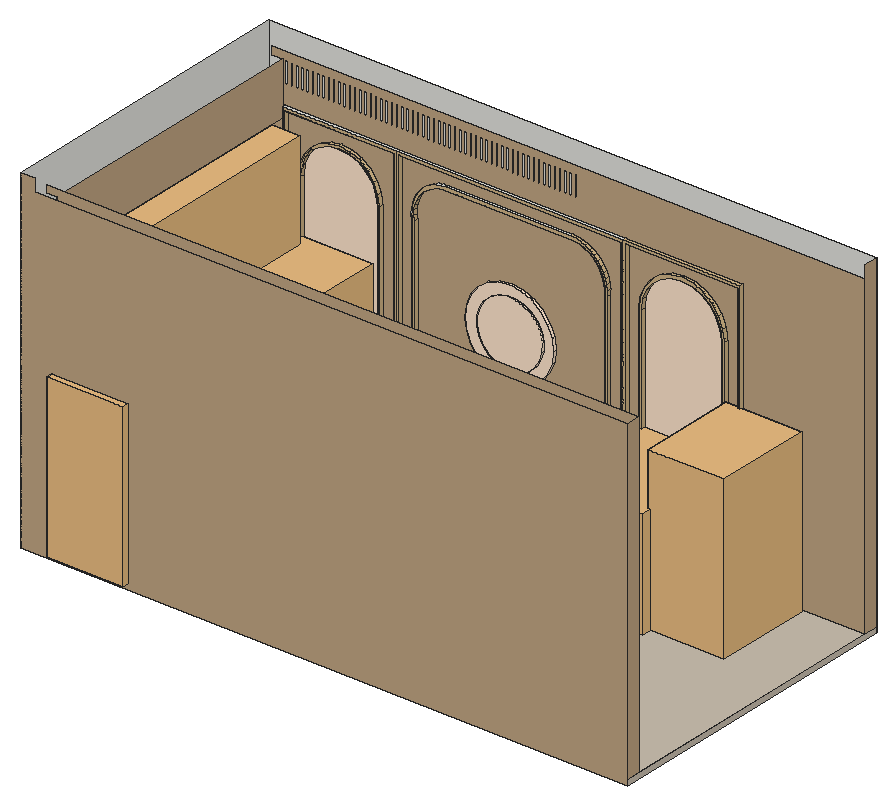
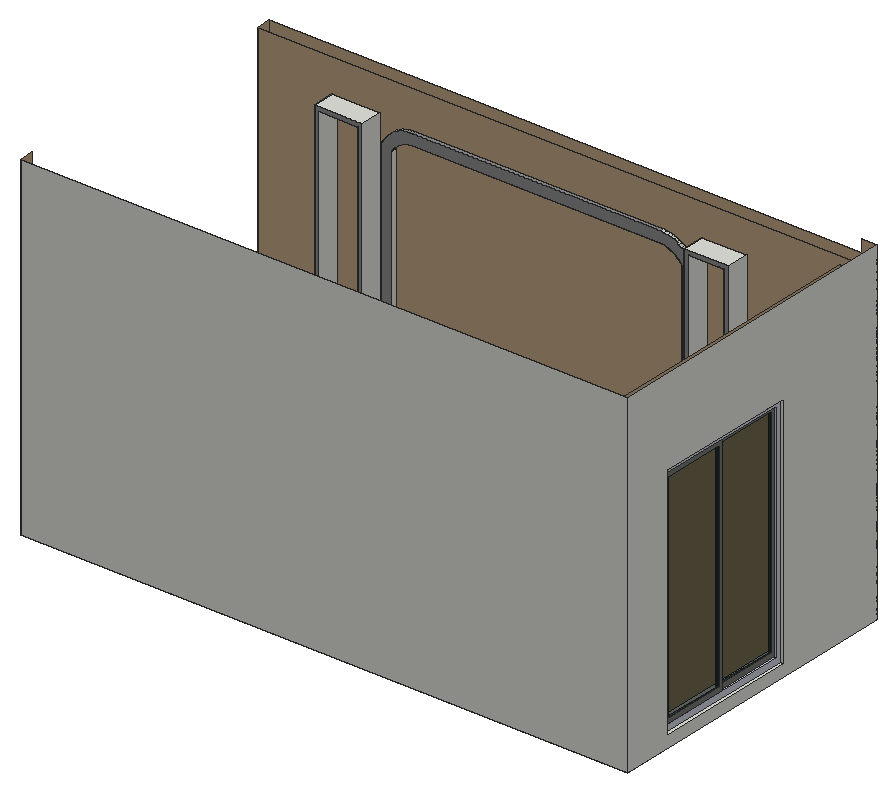
# SketchUp Ruby script. Lengths in inches.
U = 1.inch
M = Sketchup.active_model
def pt(a) = Geom::Point3d.new(a.map { |v| v * U })
def face(e, loops, mat)
  f = e.add_face(loops[0].map { |a| pt(a) })
  loops[1..].each { |l| e.add_face(l.map { |a| pt(a) }).erase! }
  f.material = f.back_material = mat if mat
  f
end
# faces: each face lists its corners as indices into pts; further lists are holes
def faces(e, pts, list, mat = nil) = list.each { |f| face(e, (f[0].is_a?(Array) ? f : [f]).map { |l| l.map { |i| pts[i] } }, mat) }
# xy, xz, yz: faces in a plane at the given z, y or x. An outline is a flat list of corners, or four numbers for a rectangle; further outlines are holes
def ring(l) = l.size == 4 ? [[l[0], l[1]], [l[2], l[1]], [l[2], l[3]], [l[0], l[3]]] : l.each_slice(2).to_a
def flat(e, list, mat, &to3) = list.each { |f| face(e, (f[0].is_a?(Array) ? f : [f]).map { |l| ring(l).map { |u, v| to3.(u, v) } }, mat) }
def xy(e, z, list, mat = nil) = flat(e, list, mat) { |x, y| [x, y, z] }
def xz(e, y, list, mat = nil) = flat(e, list, mat) { |x, z| [x, y, z] }
def yz(e, x, list, mat = nil) = flat(e, list, mat) { |y, z| [x, y, z] }
def lines(e, pts, list) = list.each { |a, b| e.add_line(pt(pts[a]), pt(pts[b])) }
# prism: a flat outline (further loops are holes) pulled along v
def prism(e, loops, v, mat = nil)
  f = face(e, loops, mat); d = Geom::Vector3d.new(v.map { |x| x * U })
  f.pushpull(f.normal.samedirection?(d) ? d.length : -d.length)
end
def box(e, o, s, mat = nil) = prism(e, [[o, [o[0] + s[0], o[1], o[2]], [o[0] + s[0], o[1] + s[1], o[2]], [o[0], o[1] + s[1], o[2]]]], [0, 0, s[2]], mat)
def at(x, y, z, deg = 0) = Geom::Transformation.translation(pt([x, y, z])) * Geom::Transformation.rotation(ORIGIN, Z_AXIS, deg.degrees)
def axes(o, x, y, z) = Geom::Transformation.new([*x, 0, *y, 0, *z, 0, *pt(o).to_a, 1])
def part(name) = M.definitions.add(name)
# library, detail: a bought-in or finely detailed component or shape, given as its bounding box
def library(name, o, s) = part(name).tap { |d| box(d.entities, o, s) }
def detail(e, o, s) = box(e.add_group.entities, o, s)
def put(e, d, t, mat = nil) = e.add_instance(d, t).tap { |i| i.material = mat if mat }
def group(e, t, mat = nil) = e.add_group.tap { |g| g.transformation = t; g.material = mat if mat }.entities
root = M.entities
M.materials.add("Maquette Wood A01 12cm").color = [209, 181, 135]
M.materials.add("Marble Beige 23-86 150cm").color = [203, 192, 176]
M.materials.add("Sand A01 200cm").color = [193, 166, 131]
M.materials.add("Wood 13-02 100cm").color = [197, 153, 102]
M.materials.add("[Color C01]").color = [255, 229, 204]
M.materials.add("[Color M04]").color = [142, 142, 142]
M.materials.add("[Metal Aluminum Anodized]").color = [202, 209, 219]
M.materials.add("[Metal Seamed]").color = [118, 119, 115]
M.materials.add("[Translucent Glass Tinted]").color = [1, 25, 30]
M.materials["[Translucent Glass Tinted]"].alpha = 0.31
c1 = library("Indoor Plant 011",[-26.56,-29.5,0],[41.02,52.38,86.8125])
c2 = library("Dome Light\#1",[-12,-12,0],[24,24,12])
c3 = library("Adapt",[-53.4375,-23.42,0],[106.875,46.86,33.24])
c4 = library("Curtains",[0,0,0],[121.73,8.19,117.22])
c5 = part("Group\#98")
g1 = group(c5.entities,at(-0.375,0,0),"[Metal Seamed]")
prism(g1,[[[0.375,0,0],[0.375,0,57],[0.375,26.94,57],[0.375,26.94,0]],[[0.375,25.82,55.875],[0.375,1.125,55.875],[0.375,1.125,1.125],[0.375,25.82,1.125]]],[1.5,0,0])
g2 = group(c5.entities,at(0.18,24.32,1.125),"[Translucent Glass Tinted]")
box(g2,[0,-23.19,0],[1.125,24.69,54.75])
c6 = part("Aluminium+Channel+Glass+Window")
g3 = group(c6.entities,at(2.67,-569.03,-1003.6875))
g4 = group(g3,at(0,0,0),"[Metal Aluminum Anodized]")
prism(g4,[[[0,0,179.5],[0,110.12,179.5],[0,110.12,0],[0,0,0]],[[0,2.9,4.49],[0,107.21,4.49],[0,107.21,175.01],[0,2.9,175.01]]],[3.86,0,0])
put(g3,c5,axes([1.96,2.9,4.49],[1.0458,0,0],[0,1.97698,0],[0,0,2.99167]))
put(g3,c5,axes([0.39,53.95,4.49],[1.0458,0,0],[0,1.97698,0],[0,0,2.99167]))
xy(root,0,[[0,0,458.14,234.875]],"Marble Beige 23-86 150cm")
xy(root,4.1875,[[135.53,10.82,354.1,14.13],[89.125,11.13,93,27.88],[93,11.13,122.82,27.88],[365.99,11.13,369.19,27.88],[369.19,11.13,401.77,27.88]])
xy(root,4.1875,[[11.13,11.13,89.125,11.13,89.125,27.88,122.82,27.88,122.82,11.13,127.25,11.13,127.25,14.13,362.38,14.13,362.38,11.13,365.99,11.13,365.99,27.88,401.77,27.88,401.77,11.13,458.14,11.13,458.14,223.75,366.32,223.75,366.32,221.18,364.32,221.18,364.32,223.75,11.13,223.75]],"Marble Beige 23-86 150cm")
xy(root,6.38,[[151.25,11.13,338.38,43.94]])
xy(root,7.64,[[93,11.13,118.94,27.88]])
xy(root,8.27,[[369.19,11.13,398.57,27.88]],"[Color M04]")
xy(root,8.75,[[0,87.63,11.13,197.75]])
xy(root,10.1875,[[20.94,221.18,104.65,223.75],[104.65,221.18,106.65,223.75],[106.65,221.18,278.07,223.75],[278.07,221.18,364.32,223.75]])
xy(root,12.1875,[[22.95,221.18,104.65,223.75],[108.65,221.18,276.07,223.75],[280.07,221.18,364.32,223.75]],"Maquette Wood A01 12cm")
xy(root,15.51,[[289.71,221.12,354.68,223.75]])
xy(root,15.77,[[118.55,221.12,266.18,223.75]])
xy(root,16.25,[[33.33,221.12,94.27,223.75]])
xy(root,17.87,[[34.95,221.12,92.65,223.75],[120.65,221.12,264.07,223.75],[292.07,221.12,352.32,223.75]],"Maquette Wood A01 12cm")
xy(root,55.53,[[151.25,11.13,338.38,43.94]],"Wood 13-02 100cm")
xy(root,188.25,[[0,87.63,11.13,197.75]])
xy(root,195.25,[[144.65,221.12,238.15,223.75]],"Maquette Wood A01 12cm")
xy(root,197.35,[[144.58,221.12,238.23,223.75]])
xy(root,198.875,[[[11.13,11.13,18.94,223.75],[12.08,12.08,18,222.8]]])
xy(root,206.4375,[[12.08,12.08,18,222.8]])
xy(root,206.625,[[22.95,221.18,104.65,223.75],[108.65,221.18,276.07,223.75],[280.07,221.18,364.32,223.75]],"Maquette Wood A01 12cm")
xy(root,207.97,[[151.81,10.82,338.18,14.13]],"[Color M04]")
xy(root,208.625,[[20.94,221.18,106.65,223.75],[106.65,221.18,278.07,223.75]])
xy(root,208.625,[[278.07,221.18,366.32,223.75]],"Maquette Wood A01 12cm")
xy(root,216.25,[[369.19,11.13,398.57,27.88]])
xy(root,216.25,[[151.25,11.13,338.38,14.13]],"[Color M04]")
xy(root,217.3125,[[93,11.13,118.94,27.88]])
xy(root,219.45,[[365.99,11.13,401.77,27.88]])
xy(root,220.13,[[89.125,11.13,122.82,27.88]])
xz(root,0,[[0,0,458.14,0,458.14,244.625,11.13,244.625,11.13,253.625,0,253.625]],"Sand A01 200cm")
xz(root,10.82,[[135.53,4.1875,135.53,198.48,136.47,199.72,137.67,201.08,138.98,202.33,140.375,203.48,141.86,204.51,143.42,205.42,145.05,206.21,146.74,206.86,148.47,207.38,150.24,207.76,151.81,207.97,338.18,207.97,340.1,207.88,341.8,207.64,343.47,207.24,345.1,206.68,346.67,205.97,348.16,205.11,349.5625,204.12,350.87,203,352.06,201.76,353.13,200.41,354.07,198.97,354.1,198.9,354.1,4.1875]],"Sand A01 200cm")
xz(root,11.13,[[89.125,0.31,122.82,4.1875],[365.99,0.99,401.77,4.1875],[151.25,6.38,338.38,55.53]])
xz(root,11.13,[[11.13,4.1875,11.13,198.875,18.94,198.875,18.94,238.625,11.13,238.625,11.13,244.625,458.14,244.625,458.14,4.1875,401.77,4.1875,401.77,219.45,365.99,219.45,365.99,4.1875,362.38,4.1875,362.38,200.9375,361.22,203.16,359.85,205.25,358.29,207.21,356.56,209.02,354.66,210.65,352.61,212.1,350.44,213.34,348.16,214.375,345.79,215.19,343.36,215.78,340.88,216.13,338.38,216.25,151.25,216.25,148.8125,215.92,146.41,215.4,144.05,214.7,141.75,213.8,139.53,212.73,137.41,211.49,135.38,210.09,133.48,208.53,131.7,206.82,130.07,204.98,128.58,203.01,127.25,200.9375,127.25,4.1875,122.82,4.1875,122.82,220.13,89.125,220.13,89.125,4.1875],[93,7.64,118.94,217.3125],[369.19,8.27,398.57,216.25]],"Sand A01 200cm")
xz(root,12.08,[[12.08,198.875,18,206.4375]])
xz(root,14.13,[[127.25,4.1875,127.25,200.9375,128.58,203.01,130.07,204.98,131.7,206.82,133.48,208.53,135.38,210.09,137.41,211.49,139.53,212.73,141.75,213.8,144.05,214.7,146.41,215.4,148.8125,215.92,151.25,216.25,338.38,216.25,340.88,216.13,343.36,215.78,345.79,215.19,348.16,214.375,350.44,213.34,352.61,212.1,354.66,210.65,356.56,209.02,358.29,207.21,359.85,205.25,361.22,203.16,362.38,200.9375,362.38,4.1875,354.1,4.1875,354.1,198.9,354.07,198.97,353.13,200.41,352.06,201.76,350.87,203,349.5625,204.12,348.16,205.11,346.67,205.97,345.1,206.68,343.47,207.24,341.8,207.64,340.1,207.88,338.18,207.97,151.81,207.97,150.24,207.76,148.47,207.38,146.74,206.86,145.05,206.21,143.42,205.42,141.86,204.51,140.375,203.48,138.98,202.33,137.67,201.08,136.47,199.72,135.53,198.48,135.53,4.1875]],"[Color M04]")
xz(root,27.88,[[[89.125,4.1875,122.82,220.13],[93,7.64,118.94,217.3125]],[[365.99,4.1875,401.77,219.45],[369.19,8.27,398.57,216.25]]],"[Color M04]")
xz(root,43.94,[[151.25,6.38,338.38,55.53]],"Wood 13-02 100cm")
xz(root,87.63,[[0,8.75,11.13,188.25]])
xz(root,197.75,[[0,8.75,11.13,188.25]])
xz(root,220.5,[[195.45,90.64,201.75,92.12,207.45,95.19,212.17,99.63,215.58,105.14,217.4375,111.35,217.63,117.82,216.15,124.125,213.08,129.83,208.64,134.54,203.125,137.95,196.92,139.8125,190.45,140.01,184.14,138.52,178.44,135.45,173.72,131.01,170.32,125.5,168.45,119.3,168.26,112.82,169.75,106.52,172.82,100.8125,177.26,96.1,182.77,92.69,188.97,90.83]],"[Color C01]")
xz(root,221.12,[[[289.71,15.51,354.68,15.51,354.68,166.4375,353.58,174.85,350.33,182.68,345.17,189.41,338.44,194.57,330.61,197.82,322.2,198.92,313.79,197.82,305.96,194.57,299.23,189.41,294.07,182.68,290.82,174.85,289.71,166.4375],[292.07,17.87,292.07,166.4375,293.1,174.23,296.11,181.5,300.9,187.74,307.14,192.53,314.4,195.54,322.2,196.5625,330,195.54,337.26,192.53,343.5,187.74,348.29,181.5,351.3,174.23,352.32,166.4375,352.32,17.87]],[[118.55,15.77,266.18,15.77,266.18,166.4,266.3125,170.15,265.9,174.06,264.96,177.875,263.48,181.52,261.52,184.93,259.1,188.03,256.27,190.76,253.09,193.07,249.62,194.92,245.92,196.27,242.08,197.09,238.23,197.35,144.58,197.35,140.79,197.08,137.02,196.24,133.4,194.86,130.03,192.96,126.97,190.6,124.28,187.82,122.03,184.67,120.26,181.23,119.01,177.57,118.3,173.77,118.16,169.9,118.55,166.32],[120.65,17.87,120.65,166.4375,120.27,169.98,120.4,173.54,121.05,177.04,122.2,180.41,123.83,183.57,125.9,186.47,128.375,189.03,131.19,191.2,134.3,192.95,137.625,194.22,141.1,194.99,144.65,195.25,238.15,195.25,241.78,195,245.34,194.24,248.76,192.99,251.97,191.29,254.91,189.15,257.53,186.62,259.77,183.75,261.59,180.6,262.95,177.22,263.83,173.69,264.2,170.07,264.07,166.4375,264.07,17.87]],[[33.33,16.25,94.27,16.25,94.27,166.4375,93.23,174.32,90.19,181.67,85.35,187.98,79.04,192.82,71.6875,195.87,63.8,196.91,55.92,195.87,48.57,192.82,42.26,187.98,37.42,181.67,34.37,174.32,33.33,166.4375],[34.95,17.87,34.95,166.4375,35.9375,173.9,38.82,180.86,43.4,186.84,49.38,191.42,56.34,194.3,63.8,195.29,71.27,194.3,78.23,191.42,84.2,186.84,88.79,180.86,91.67,173.9,92.65,166.4375,92.65,17.87]]],"Maquette Wood A01 12cm")
xz(root,221.18,[[364.32,4.1875,366.32,4.1875,366.32,208.625,278.07,208.625,278.07,10.1875,364.32,10.1875,364.32,12.1875,280.07,12.1875,280.07,206.625,364.32,206.625],[[20.94,10.1875,106.65,208.625],[22.95,12.1875,104.65,206.625]],[[106.65,10.1875,278.07,208.625],[108.65,12.1875,276.07,206.625]]],"Maquette Wood A01 12cm")
xz(root,221.93,[[[191.72,80.375,200.45,81.53,208.59,84.9,215.58,90.26,220.94,97.25,224.32,105.39,225.47,114.125,224.32,122.86,220.94,131,215.58,137.99,208.59,143.35,200.45,146.72,191.72,147.875,182.98,146.72,174.84,143.35,167.85,137.99,162.49,131,159.12,122.86,157.97,114.125,159.12,105.39,162.49,97.25,167.85,90.26,174.84,84.9,182.98,81.53],[195.45,90.64,188.97,90.83,182.77,92.69,177.26,96.1,172.82,100.8125,169.75,106.52,168.26,112.82,168.45,119.3,170.32,125.5,173.72,131.01,178.44,135.45,184.14,138.52,190.45,140.01,196.92,139.8125,203.125,137.95,208.64,134.54,213.08,129.83,216.15,124.125,217.63,117.82,217.4375,111.35,215.58,105.14,212.17,99.63,207.45,95.19,201.75,92.12]]],"[Color C01]")
xz(root,222.8,[[12.08,198.875,18,206.4375]])
xz(root,223.75,[[[11.13,4.1875,364.32,4.1875,364.32,10.1875,20.94,10.1875,20.94,208.625,366.32,208.625,366.32,4.1875,458.14,4.1875,458.14,244.625,11.13,244.625,11.13,238.625,18.94,238.625,18.94,198.875,11.13,198.875],[56.67,222.8125,58.61,238.625],[60.64,222.8125,62.58,238.625],[64.6,222.8125,66.55,238.625],[68.57,222.8125,70.52,238.625],[72.54,222.8125,74.49,238.625],[76.51,222.8125,78.45,238.625],[80.48,222.8125,82.42,238.625],[84.45,222.8125,86.39,238.625],[88.42,222.8125,90.36,238.625],[92.39,222.8125,94.33,238.625],[96.36,222.8125,98.3,238.625],[100.33,222.8125,102.27,238.625],[104.3,222.8125,106.24,238.625],[108.27,222.8125,110.21,238.625],[112.24,222.8125,114.18,238.625],[116.21,222.8125,118.15,238.625],[120.18,222.8125,122.12,238.625],[124.14,222.8125,126.09,238.625],[20.94,222.8125,22.88,238.625],[24.91,222.8125,26.85,238.625],[28.88,222.8125,30.82,238.625],[32.85,222.8125,34.79,238.625],[36.82,222.8125,38.76,238.625],[40.79,222.8125,42.73,238.625],[44.76,222.8125,46.7,238.625],[48.73,222.8125,50.67,238.625],[52.7,222.8125,54.64,238.625],[128.11,222.8125,130.06,238.625],[132.08,222.8125,134.03,238.625],[136.05,222.8125,137.99,238.625],[140.02,222.8125,141.96,238.625],[143.99,222.8125,145.93,238.625],[147.96,222.8125,149.9,238.625],[151.93,222.8125,153.87,238.625],[155.9,222.8125,157.84,238.625],[159.87,222.8125,161.81,238.625],[163.84,222.8125,165.78,238.625],[167.81,222.8125,169.75,238.625],[171.78,222.8125,173.72,238.625],[175.75,222.8125,177.6875,238.625],[179.71,222.8125,181.66,238.625],[183.68,222.8125,185.625,238.625],[187.65,222.8125,189.6,238.625],[191.62,222.8125,193.56,238.625],[195.59,222.8125,197.53,238.625],[199.5625,222.8125,201.5,238.625],[203.53,222.8125,205.47,238.625],[207.5,222.8125,209.44,238.625],[211.47,222.8125,213.41,238.625],[215.4375,222.8125,217.38,238.625],[219.41,222.8125,221.35,238.625],[223.38,222.8125,225.32,238.625],[227.35,222.8125,229.29,238.625],[231.32,222.8125,233.26,238.625],[235.29,222.8125,237.23,238.625],[239.25,222.8125,241.2,238.625]],[[22.95,12.1875,104.65,206.625],[33.33,16.25,33.33,166.4375,34.37,174.32,37.42,181.67,42.26,187.98,48.57,192.82,55.92,195.87,63.8,196.91,71.6875,195.87,79.04,192.82,85.35,187.98,90.19,181.67,93.23,174.32,94.27,166.4375,94.27,16.25]],[[108.65,12.1875,276.07,206.625],[118.55,15.77,118.55,166.32,118.16,169.9,118.3,173.77,119.01,177.57,120.26,181.23,122.03,184.67,124.28,187.82,126.97,190.6,130.03,192.96,133.4,194.86,137.02,196.24,140.79,197.08,144.58,197.35,238.23,197.35,242.08,197.09,245.92,196.27,249.62,194.92,253.09,193.07,256.27,190.76,259.1,188.03,261.52,184.93,263.48,181.52,264.96,177.875,265.9,174.06,266.3125,170.15,266.18,166.4,266.18,15.77]],[[280.07,12.1875,364.32,206.625],[289.71,15.51,289.71,166.4375,290.82,174.85,294.07,182.68,299.23,189.41,305.96,194.57,313.79,197.82,322.2,198.92,330.61,197.82,338.44,194.57,345.17,189.41,350.33,182.68,353.58,174.85,354.68,166.4375,354.68,15.51]],[[120.65,17.87,264.07,17.87,264.07,166.4375,264.2,170.07,263.83,173.69,262.95,177.22,261.59,180.6,259.77,183.75,257.53,186.62,254.91,189.15,251.97,191.29,248.76,192.99,245.34,194.24,241.78,195,238.15,195.25,144.65,195.25,141.1,194.99,137.625,194.22,134.3,192.95,131.19,191.2,128.375,189.03,125.9,186.47,123.83,183.57,122.2,180.41,121.05,177.04,120.4,173.54,120.27,169.98,120.65,166.4375],[191.72,80.375,182.98,81.53,174.84,84.9,167.85,90.26,162.49,97.25,159.12,105.39,157.97,114.125,159.12,122.86,162.49,131,167.85,137.99,174.84,143.35,182.98,146.72,191.72,147.875,200.45,146.72,208.59,143.35,215.58,137.99,220.94,131,224.32,122.86,225.47,114.125,224.32,105.39,220.94,97.25,215.58,90.26,208.59,84.9,200.45,81.53]]],"Sand A01 200cm")
xz(root,223.75,[[34.95,17.87,92.65,17.87,92.65,166.4375,91.67,173.9,88.79,180.86,84.2,186.84,78.23,191.42,71.27,194.3,63.8,195.29,56.34,194.3,49.38,191.42,43.4,186.84,38.82,180.86,35.9375,173.9,34.95,166.4375],[292.07,17.87,352.32,17.87,352.32,166.4375,351.3,174.23,348.29,181.5,343.5,187.74,337.26,192.53,330,195.54,322.2,196.5625,314.4,195.54,307.14,192.53,300.9,187.74,296.11,181.5,293.1,174.23,292.07,166.4375]],"[Color C01]")
xz(root,234.875,[[0,0,458.14,253.625]])
yz(root,0,[[[0,0,234.875,253.625],[87.63,8.75,197.75,188.25]]])
yz(root,11.13,[[[11.13,4.1875,223.75,198.875],[87.63,8.75,197.75,188.25]]],"Sand A01 200cm")
yz(root,12.08,[[12.08,198.875,222.8,206.4375]])
yz(root,18,[[12.08,198.875,222.8,206.4375]])
yz(root,18.94,[[11.13,198.875,223.75,238.625]],"Sand A01 200cm")
yz(root,20.94,[[221.18,10.1875,223.75,208.625]])
yz(root,22.95,[[221.18,12.1875,223.75,206.625]],"Maquette Wood A01 12cm")
yz(root,33.33,[[221.12,16.25,223.75,166.4375]])
yz(root,34.95,[[221.12,17.87,223.75,166.4375]],"Maquette Wood A01 12cm")
yz(root,89.125,[[11.13,4.1875,27.88,220.13]])
yz(root,92.65,[[221.12,17.87,223.75,166.4375]],"Maquette Wood A01 12cm")
yz(root,93,[[11.13,7.64,27.88,217.3125]],"[Color M04]")
yz(root,94.27,[[221.12,16.25,223.75,166.4375]],"Maquette Wood A01 12cm")
yz(root,104.65,[[221.18,12.1875,223.75,206.625]],"Maquette Wood A01 12cm")
yz(root,108.65,[[221.18,12.1875,223.75,206.625]],"Maquette Wood A01 12cm")
yz(root,118.55,[[221.12,15.77,223.75,166.32]])
yz(root,118.94,[[11.13,7.64,27.88,217.3125]])
yz(root,120.65,[[221.12,17.87,223.75,166.4375]],"Maquette Wood A01 12cm")
yz(root,122.82,[[11.13,4.1875,27.88,220.13]],"[Color M04]")
yz(root,127.25,[[11.13,4.1875,14.13,200.9375]])
yz(root,135.53,[[10.82,4.1875,14.13,198.48]],"[Color M04]")
yz(root,151.25,[[11.13,6.38,43.94,55.53]],"Wood 13-02 100cm")
yz(root,264.07,[[221.12,17.87,223.75,166.4375]])
yz(root,266.18,[[221.12,15.77,223.75,166.4]],"Maquette Wood A01 12cm")
yz(root,276.07,[[221.18,12.1875,223.75,206.625]],"Maquette Wood A01 12cm")
yz(root,280.07,[[221.18,12.1875,223.75,206.625]],"Maquette Wood A01 12cm")
yz(root,289.71,[[221.12,15.51,223.75,166.4375]],"Maquette Wood A01 12cm")
yz(root,292.07,[[221.12,17.87,223.75,166.4375]],"Maquette Wood A01 12cm")
yz(root,338.38,[[11.13,6.38,43.94,55.53]],"Wood 13-02 100cm")
yz(root,352.32,[[221.12,17.87,223.75,166.4375]],"Maquette Wood A01 12cm")
yz(root,354.1,[[10.82,4.1875,14.13,198.9]])
yz(root,354.68,[[221.12,15.51,223.75,166.4375]],"Maquette Wood A01 12cm")
yz(root,362.38,[[11.13,4.1875,14.13,200.9375]])
yz(root,364.32,[[221.18,4.1875,223.75,10.1875],[221.18,10.1875,223.75,12.1875]])
yz(root,364.32,[[221.18,12.1875,223.75,206.625]],"Maquette Wood A01 12cm")
yz(root,365.99,[[11.13,4.1875,27.88,219.45]])
yz(root,366.32,[[221.18,4.1875,223.75,208.625]],"Maquette Wood A01 12cm")
yz(root,369.19,[[11.13,8.27,27.88,216.25]],"[Color M04]")
yz(root,398.57,[[11.13,8.27,27.88,216.25]])
yz(root,401.77,[[11.13,4.1875,27.88,219.45]],"[Color M04]")
yz(root,458.14,[[0,0,234.875,4.1875]],"Marble Beige 23-86 150cm")
yz(root,458.14,[[0,4.1875,11.13,244.625],[223.75,4.1875,234.875,253.625]],"Sand A01 200cm")
p = [[182.98,223.75,81.53],[191.72,223.75,80.375],[191.72,221.93,80.375],[182.98,221.93,81.53],[200.45,223.75,81.53],[200.45,221.93,81.53],
  [174.84,223.75,84.9],[174.84,221.93,84.9],[208.59,223.75,84.9],[208.59,221.93,84.9],[167.85,223.75,90.26],[167.85,221.93,90.26],
  [215.58,223.75,90.26],[215.58,221.93,90.26],[162.49,223.75,97.25],[162.49,221.93,97.25],[220.94,223.75,97.25],[220.94,221.93,97.25],
  [188.97,221.93,90.83],[195.45,221.93,90.64],[195.45,220.5,90.64],[188.97,220.5,90.83],[201.75,221.93,92.12],[201.75,220.5,92.12],
  [182.77,221.93,92.69],[182.77,220.5,92.69],[207.45,221.93,95.19],[207.45,220.5,95.19],[177.26,221.93,96.1],[177.26,220.5,96.1],
  [212.17,221.93,99.63],[212.17,220.5,99.63],[172.82,221.93,100.8125],[172.82,220.5,100.8125],[159.12,223.75,105.39],[159.12,221.93,105.39],
  [224.32,223.75,105.39],[224.32,221.93,105.39],[215.58,221.93,105.14],[215.58,220.5,105.14],[169.75,221.93,106.52],[169.75,220.5,106.52],
  [217.4375,221.93,111.35],[217.4375,220.5,111.35],[157.97,223.75,114.125],[157.97,221.93,114.125],[225.47,223.75,114.125],[225.47,221.93,114.125],
  [168.26,221.93,112.82],[168.26,220.5,112.82],[217.63,221.93,117.82],[217.63,220.5,117.82],[168.45,221.93,119.3],[168.45,220.5,119.3],
  [159.12,223.75,122.86],[159.12,221.93,122.86],[224.32,223.75,122.86],[224.32,221.93,122.86],[216.15,221.93,124.125],[216.15,220.5,124.125],
  [170.32,221.93,125.5],[170.32,220.5,125.5],[162.49,223.75,131],[162.49,221.93,131],[220.94,223.75,131],[220.94,221.93,131],
  [213.08,221.93,129.83],[213.08,220.5,129.83],[173.72,221.93,131.01],[173.72,220.5,131.01],[208.64,221.93,134.54],[208.64,220.5,134.54],
  [178.44,221.93,135.45],[178.44,220.5,135.45],[167.85,223.75,137.99],[167.85,221.93,137.99],[215.58,223.75,137.99],[215.58,221.93,137.99],
  [203.125,221.93,137.95],[203.125,220.5,137.95],[184.14,221.93,138.52],[184.14,220.5,138.52],[196.92,221.93,139.8125],[196.92,220.5,139.8125],
  [174.84,223.75,143.35],[174.84,221.93,143.35],[208.59,223.75,143.35],[208.59,221.93,143.35],[190.45,221.93,140.01],[190.45,220.5,140.01],
  [182.98,223.75,146.72],[182.98,221.93,146.72],[200.45,223.75,146.72],[200.45,221.93,146.72],[191.72,223.75,147.875],[191.72,221.93,147.875],
  [118.16,223.75,169.9],[118.55,223.75,166.32],[118.55,221.12,166.32],[118.16,221.12,169.9],[34.37,223.75,174.32],[33.33,223.75,166.4375],
  [33.33,221.12,166.4375],[34.37,221.12,174.32],[34.95,223.75,166.4375],[35.9375,223.75,173.9],[35.9375,221.12,173.9],[34.95,221.12,166.4375],
  [91.67,223.75,173.9],[92.65,223.75,166.4375],[92.65,221.12,166.4375],[91.67,221.12,173.9],[94.27,223.75,166.4375],[93.23,223.75,174.32],
  [93.23,221.12,174.32],[94.27,221.12,166.4375],[120.65,223.75,166.4375],[120.27,223.75,169.98],[120.27,221.12,169.98],[120.65,221.12,166.4375],
  [264.2,223.75,170.07],[264.07,223.75,166.4375],[264.07,221.12,166.4375],[264.2,221.12,170.07],[266.18,223.75,166.4],[266.3125,223.75,170.15],
  [266.3125,221.12,170.15],[266.18,221.12,166.4],[290.82,223.75,174.85],[289.71,223.75,166.4375],[289.71,221.12,166.4375],[290.82,221.12,174.85],
  [292.07,223.75,166.4375],[293.1,223.75,174.23],[293.1,221.12,174.23],[292.07,221.12,166.4375],[351.3,223.75,174.23],[352.32,223.75,166.4375],
  [352.32,221.12,166.4375],[351.3,221.12,174.23],[354.68,223.75,166.4375],[353.58,223.75,174.85],[353.58,221.12,174.85],[354.68,221.12,166.4375],
  [118.3,223.75,173.77],[118.3,221.12,173.77],[120.4,223.75,173.54],[120.4,221.12,173.54],[263.83,223.75,173.69],[263.83,221.12,173.69],
  [265.9,223.75,174.06],[265.9,221.12,174.06],[121.05,223.75,177.04],[121.05,221.12,177.04],[262.95,223.75,177.22],[262.95,221.12,177.22],
  [119.01,223.75,177.57],[119.01,221.12,177.57],[38.82,223.75,180.86],[38.82,221.12,180.86],[88.79,223.75,180.86],[88.79,221.12,180.86],
  [264.96,223.75,177.875],[264.96,221.12,177.875],[296.11,223.75,181.5],[296.11,221.12,181.5],[348.29,223.75,181.5],[348.29,221.12,181.5],
  [37.42,223.75,181.67],[37.42,221.12,181.67],[90.19,223.75,181.67],[90.19,221.12,181.67],[294.07,223.75,182.68],[294.07,221.12,182.68],
  [350.33,223.75,182.68],[350.33,221.12,182.68],[122.2,223.75,180.41],[122.2,221.12,180.41],[261.59,223.75,180.6],[261.59,221.12,180.6],
  [120.26,223.75,181.23],[120.26,221.12,181.23],[263.48,223.75,181.52],[263.48,221.12,181.52],[123.83,223.75,183.57],[123.83,221.12,183.57],
  [259.77,223.75,183.75],[259.77,221.12,183.75],[43.4,223.75,186.84],[43.4,221.12,186.84],[84.2,223.75,186.84],[84.2,221.12,186.84],
  [122.03,223.75,184.67],[122.03,221.12,184.67],[261.52,223.75,184.93],[261.52,221.12,184.93],[300.9,223.75,187.74],[300.9,221.12,187.74],
  [343.5,223.75,187.74],[343.5,221.12,187.74],[42.26,223.75,187.98],[42.26,221.12,187.98],[85.35,223.75,187.98],[85.35,221.12,187.98],
  [299.23,223.75,189.41],[299.23,221.12,189.41],[345.17,223.75,189.41],[345.17,221.12,189.41],[125.9,223.75,186.47],[125.9,221.12,186.47],
  [257.53,223.75,186.62],[257.53,221.12,186.62],[124.28,223.75,187.82],[124.28,221.12,187.82],[259.1,223.75,188.03],[259.1,221.12,188.03],
  [128.375,223.75,189.03],[128.375,221.12,189.03],[254.91,223.75,189.15],[254.91,221.12,189.15],[49.38,223.75,191.42],[49.38,221.12,191.42],
  [78.23,223.75,191.42],[78.23,221.12,191.42],[307.14,223.75,192.53],[307.14,221.12,192.53],[337.26,223.75,192.53],[337.26,221.12,192.53],
  [126.97,223.75,190.6],[126.97,221.12,190.6],[48.57,223.75,192.82],[48.57,221.12,192.82],[79.04,223.75,192.82],[79.04,221.12,192.82],
  [256.27,223.75,190.76],[256.27,221.12,190.76],[131.19,223.75,191.2],[131.19,221.12,191.2],[251.97,223.75,191.29],[251.97,221.12,191.29],
  [305.96,223.75,194.57],[305.96,221.12,194.57],[338.44,223.75,194.57],[338.44,221.12,194.57],[130.03,223.75,192.96],[130.03,221.12,192.96],
  [253.09,223.75,193.07],[253.09,221.12,193.07],[134.3,223.75,192.95],[134.3,221.12,192.95],[248.76,223.75,192.99],[248.76,221.12,192.99],
  [56.34,223.75,194.3],[56.34,221.12,194.3],[71.27,223.75,194.3],[71.27,221.12,194.3],[314.4,223.75,195.54],[314.4,221.12,195.54],
  [330,223.75,195.54],[330,221.12,195.54],[55.92,223.75,195.87],[55.92,221.12,195.87],[71.6875,223.75,195.87],[71.6875,221.12,195.87],
  [137.625,223.75,194.22],[137.625,221.12,194.22],[133.4,223.75,194.86],[133.4,221.12,194.86],[245.34,223.75,194.24],[245.34,221.12,194.24],
  [249.62,223.75,194.92],[249.62,221.12,194.92],[141.1,223.75,194.99],[141.1,221.12,194.99],[241.78,223.75,195],[241.78,221.12,195],
  [63.8,223.75,195.29],[63.8,221.12,195.29],[313.79,223.75,197.82],[313.79,221.12,197.82],[330.61,223.75,197.82],[330.61,221.12,197.82],
  [137.02,223.75,196.24],[137.02,221.12,196.24],[245.92,223.75,196.27],[245.92,221.12,196.27],[144.65,223.75,195.25],[144.65,221.12,195.25],
  [238.15,223.75,195.25],[238.15,221.12,195.25],[322.2,223.75,196.5625],[322.2,221.12,196.5625],[63.8,223.75,196.91],[63.8,221.12,196.91],
  [140.79,223.75,197.08],[140.79,221.12,197.08],[242.08,223.75,197.09],[242.08,221.12,197.09],[144.58,223.75,197.35],[144.58,221.12,197.35],
  [238.23,223.75,197.35],[238.23,221.12,197.35],[322.2,223.75,198.92],[322.2,221.12,198.92],[135.53,14.13,198.48],[136.47,14.13,199.72],
  [136.47,10.82,199.72],[135.53,10.82,198.48],[354.07,14.13,198.97],[354.1,14.13,198.9],[354.1,10.82,198.9],[354.07,10.82,198.97],
  [353.13,14.13,200.41],[353.13,10.82,200.41],[137.67,14.13,201.08],[137.67,10.82,201.08],[352.06,14.13,201.76],[352.06,10.82,201.76],
  [127.25,11.13,200.9375],[128.58,11.13,203.01],[128.58,14.13,203.01],[127.25,14.13,200.9375],[361.22,11.13,203.16],[362.38,11.13,200.9375],
  [362.38,14.13,200.9375],[361.22,14.13,203.16],[138.98,14.13,202.33],[138.98,10.82,202.33],[350.87,14.13,203],[350.87,10.82,203],
  [140.375,14.13,203.48],[140.375,10.82,203.48],[349.5625,14.13,204.12],[349.5625,10.82,204.12],[130.07,11.13,204.98],[130.07,14.13,204.98],
  [359.85,11.13,205.25],[359.85,14.13,205.25],[141.86,14.13,204.51],[141.86,10.82,204.51],[348.16,14.13,205.11],[348.16,10.82,205.11],
  [143.42,14.13,205.42],[143.42,10.82,205.42],[131.7,11.13,206.82],[131.7,14.13,206.82],[346.67,14.13,205.97],[346.67,10.82,205.97],
  [358.29,11.13,207.21],[358.29,14.13,207.21],[145.05,14.13,206.21],[145.05,10.82,206.21],[345.1,14.13,206.68],[345.1,10.82,206.68],
  [146.74,14.13,206.86],[146.74,10.82,206.86],[343.47,14.13,207.24],[343.47,10.82,207.24],[133.48,11.13,208.53],[133.48,14.13,208.53],
  [148.47,14.13,207.38],[148.47,10.82,207.38],[341.8,14.13,207.64],[341.8,10.82,207.64],[356.56,11.13,209.02],[356.56,14.13,209.02],
  [150.24,14.13,207.76],[150.24,10.82,207.76],[340.1,14.13,207.88],[340.1,10.82,207.88],[151.81,14.13,207.97],[151.81,10.82,207.97],
  [338.18,14.13,207.97],[338.18,10.82,207.97],[135.38,11.13,210.09],[135.38,14.13,210.09],[354.66,11.13,210.65],[354.66,14.13,210.65],
  [137.41,11.13,211.49],[137.41,14.13,211.49],[352.61,11.13,212.1],[352.61,14.13,212.1],[139.53,11.13,212.73],[139.53,14.13,212.73],
  [350.44,11.13,213.34],[350.44,14.13,213.34],[141.75,11.13,213.8],[141.75,14.13,213.8],[348.16,11.13,214.375],[348.16,14.13,214.375],
  [144.05,11.13,214.7],[144.05,14.13,214.7],[345.79,11.13,215.19],[345.79,14.13,215.19],[146.41,11.13,215.4],[146.41,14.13,215.4],
  [343.36,11.13,215.78],[343.36,14.13,215.78],[148.8125,11.13,215.92],[148.8125,14.13,215.92],[340.88,11.13,216.13],[340.88,14.13,216.13],
  [151.25,11.13,216.25],[151.25,14.13,216.25],[338.38,11.13,216.25],[338.38,14.13,216.25]]
faces(root,p,[[0,1,2,3],[1,4,5,2],[6,0,3,7],[4,8,9,5],[10,6,7,11],[8,12,13,9],[14,10,11,15],[12,16,17,13],
  [18,19,20,21],[19,22,23,20],[24,18,21,25],[22,26,27,23],[28,24,25,29],[26,30,31,27],[32,28,29,33],[34,14,15,35],
  [16,36,37,17],[30,38,39,31],[40,32,33,41],[38,42,43,39],[44,34,35,45],[36,46,47,37],[48,40,41,49],[42,50,51,43],
  [52,48,49,53],[54,44,45,55],[46,56,57,47],[50,58,59,51],[60,52,53,61],[62,54,55,63],[56,64,65,57],[58,66,67,59],
  [68,60,61,69],[66,70,71,67],[72,68,69,73],[74,62,63,75],[64,76,77,65],[70,78,79,71],[80,72,73,81],[78,82,83,79],
  [84,74,75,85],[76,86,87,77],[88,80,81,89],[82,88,89,83],[90,84,85,91],[86,92,93,87],[94,90,91,95],[92,94,95,93]],"[Color C01]")
faces(root,p,[[96,97,98,99],[144,96,99,145],[156,144,145,157],[180,156,157,181],[192,180,181,193],[212,192,193,213],[228,212,213,229],[244,228,229,245],
  [266,244,245,267],[282,266,267,283],[294,282,283,295],[298,294,295,299],[318,319,320,321],[319,334,335,320],[334,344,345,335],[344,358,359,345],
  [358,374,375,359],[374,378,379,375],[378,382,383,379],[382,386,387,383],[386,390,391,387],[390,394,395,391],[394,398,399,395],[398,402,403,399]])
faces(root,p,[[100,101,102,103],[104,105,106,107],[108,109,110,111],[112,113,114,115],[116,117,118,119],[120,121,122,123],[124,125,126,127],[128,129,130,131],
  [132,133,134,135],[136,137,138,139],[140,141,142,143],[117,146,147,118],[148,120,123,149],[125,150,151,126],[146,152,153,147],[154,148,149,155],
  [105,158,159,106],[160,108,111,161],[150,162,163,151],[133,164,165,134],[166,136,139,167],[168,100,103,169],[113,170,171,114],[172,128,131,173],
  [141,174,175,142],[152,176,177,153],[178,154,155,179],[162,182,183,163],[176,184,185,177],[186,178,179,187],[158,188,189,159],[190,160,161,191],
  [182,194,195,183],[164,196,197,165],[198,166,167,199],[200,168,169,201],[170,202,203,171],[204,172,173,205],[174,206,207,175],[184,208,209,185],
  [210,186,187,211],[194,214,215,195],[208,216,217,209],[218,210,211,219],[188,220,221,189],[222,190,191,223],[196,224,225,197],[226,198,199,227],
  [230,200,201,231],[202,232,233,203],[214,234,235,215],[216,236,237,217],[238,218,219,239],[240,204,205,241],[206,242,243,207],[234,246,247,235],
  [236,248,249,237],[250,238,239,251],[220,252,253,221],[254,222,223,255],[224,256,257,225],[258,226,227,259],[260,230,231,261],[232,262,263,233],
  [248,264,265,249],[268,250,251,269],[246,270,271,247],[264,272,273,265],[274,268,269,275],[252,276,277,253],[276,254,255,277],[278,240,241,279],
  [242,280,281,243],[270,284,285,271],[272,286,287,273],[288,274,275,289],[256,290,291,257],[290,258,259,291],[292,260,261,293],[262,292,293,263],
  [284,296,297,285],[296,300,301,297],[302,278,279,303],[280,302,303,281]],"Maquette Wood A01 12cm")
faces(root,p,[[304,305,306,307],[308,309,310,311],[312,308,311,313],[305,314,315,306],[316,312,313,317],[322,323,324,325],[314,326,327,315],[328,316,317,329],
  [326,330,331,327],[332,328,329,333],[336,322,325,337],[330,338,339,331],[340,332,333,341],[338,342,343,339],[346,340,341,347],[348,336,337,349],
  [342,350,351,343],[352,346,347,353],[350,354,355,351],[356,352,353,357],[354,360,361,355],[362,356,357,363],[364,348,349,365],[360,366,367,361],
  [368,362,363,369],[366,370,371,367],[372,368,369,373],[376,364,365,377],[380,376,377,381],[384,380,381,385],[388,384,385,389],[392,388,389,393],
  [396,392,393,397],[400,396,397,401],[404,400,401,405]],"[Color M04]")
put(root,c1,axes([67.99,189.93,4.1875],[1.4,0,0],[0,1.4,0],[0,0,1.4]))
put(root,c1,axes([391.93,189.93,4.1875],[1.4,0,0],[0,1.4,0],[0,0,1.4]))
put(root,c2,axes([174.25,98.67,4.1875],[1,0,0],[0,1.43,0],[0,0,2.43]))
put(root,c3,axes([241.77,182.97,4.1875],[2.14775,0,0],[0,1.775,0],[0,0,2.46725]))
put(root,c1,axes([61.14,36.5,4.44],[1.4,0,0],[0,1.4,0],[0,0,1.4]))
put(root,c4,axes([18.94,213.68,6.65],[0,-1.63147,0],[2.58,0,0],[0,0,1.63988]))
put(root,c6,at(0,656.66,1012.4375))
